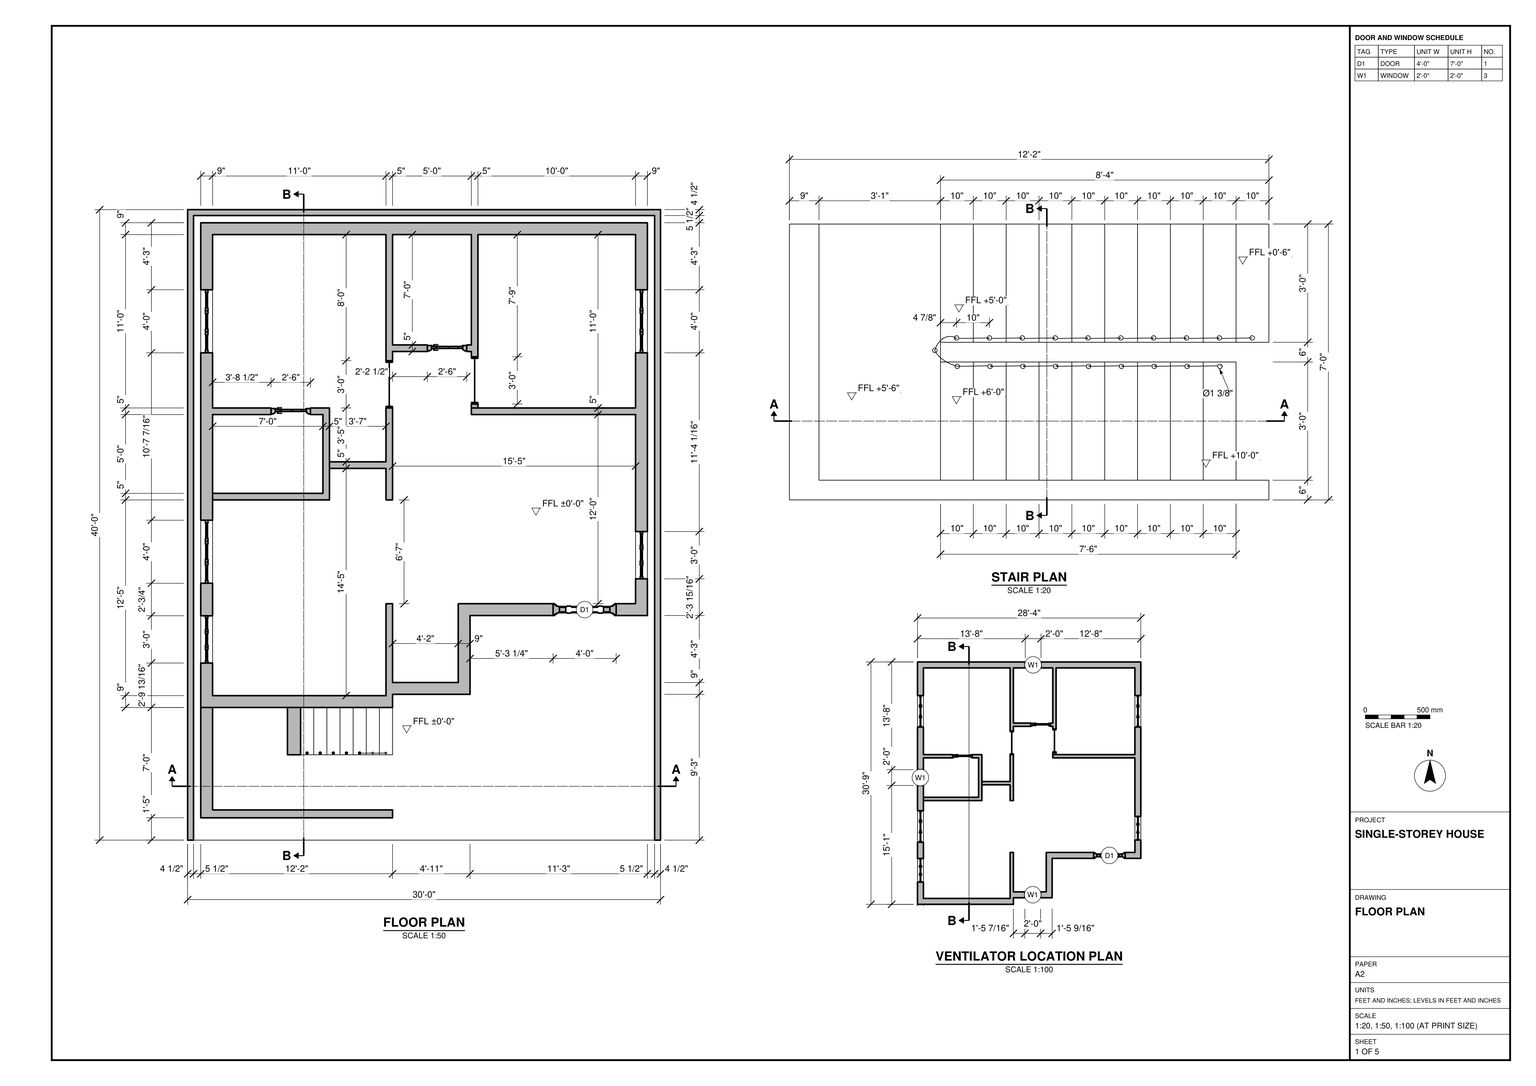
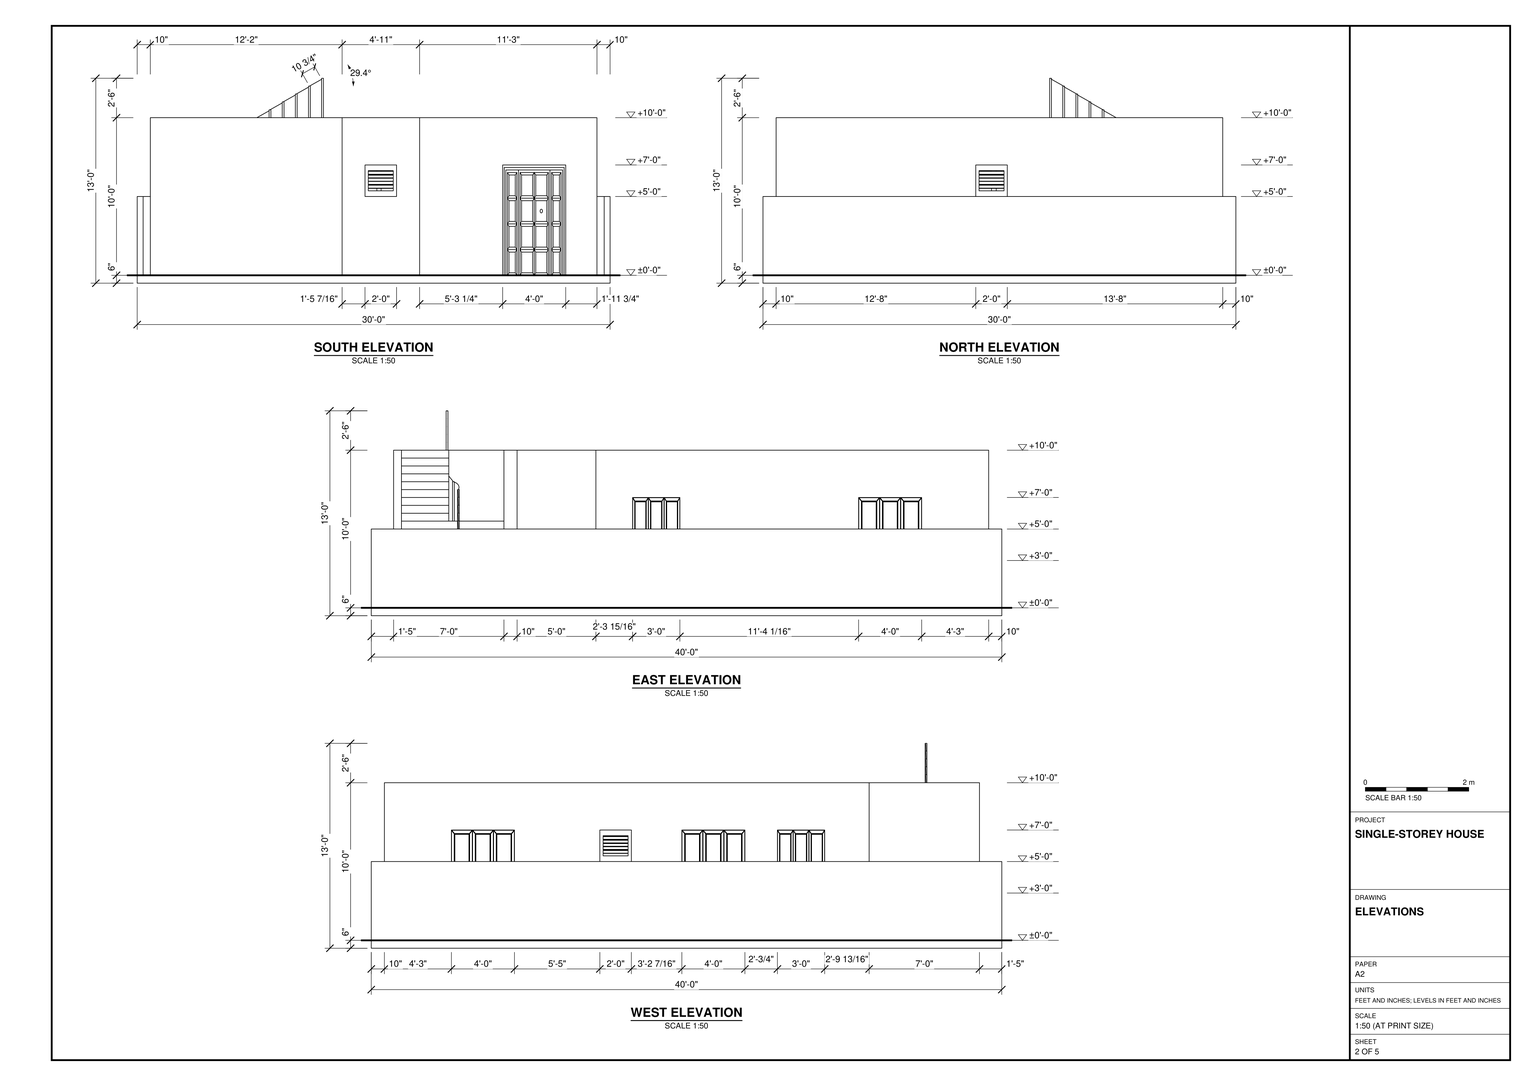
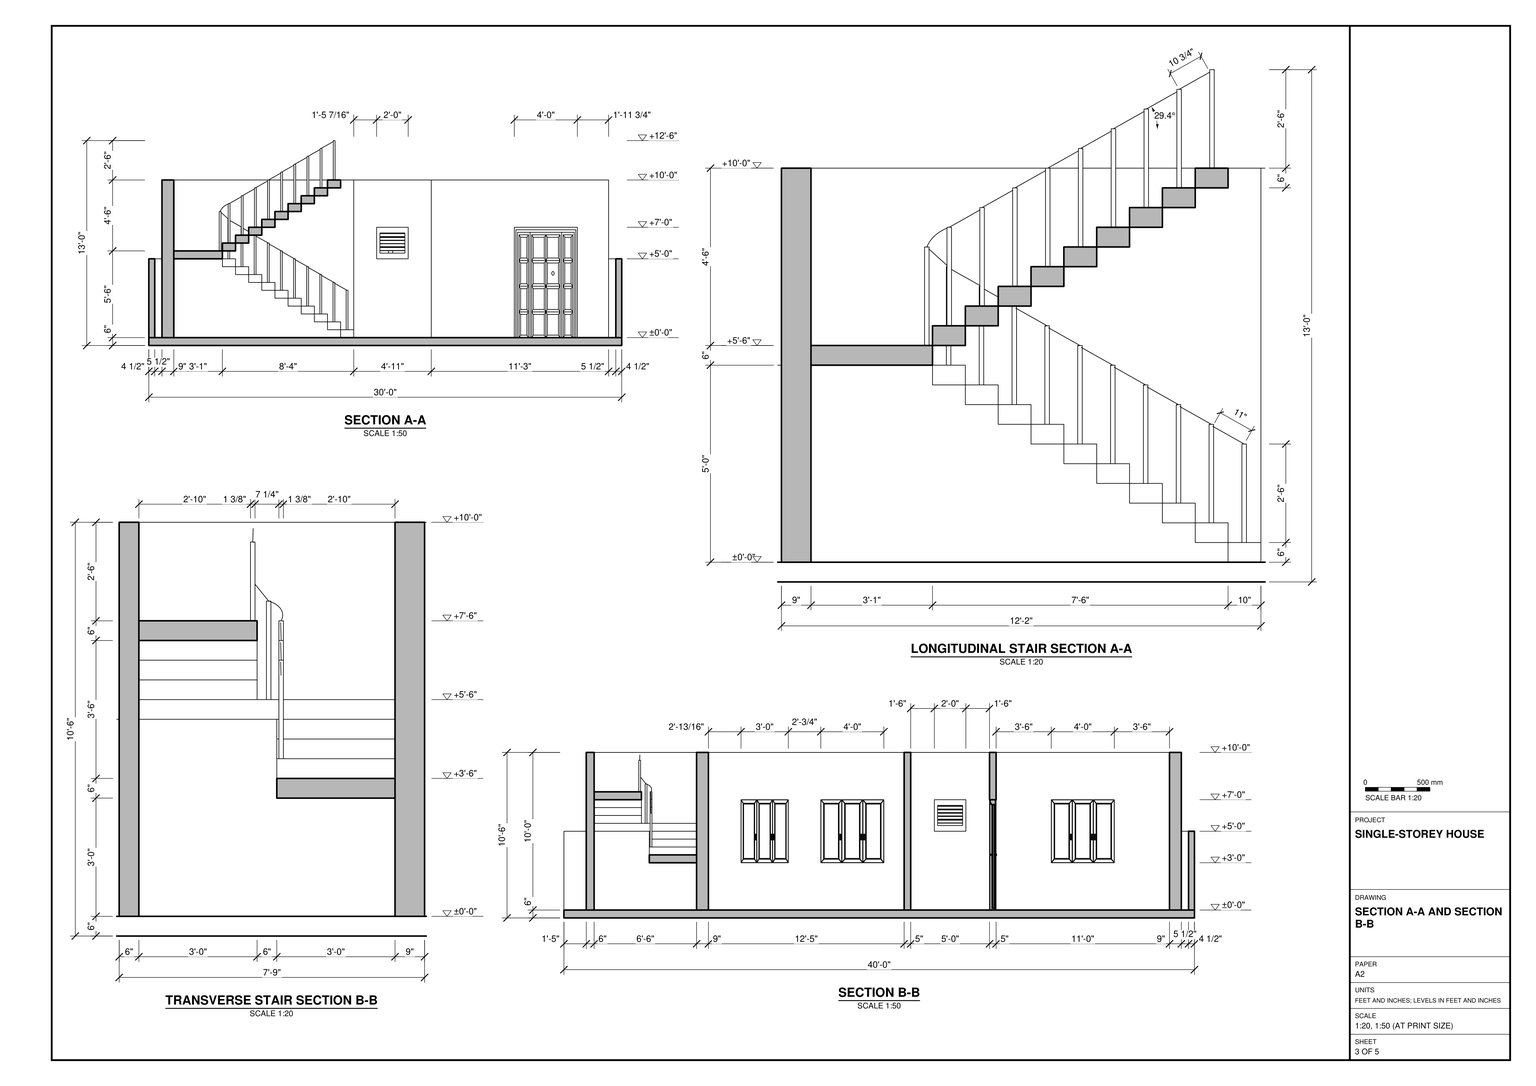
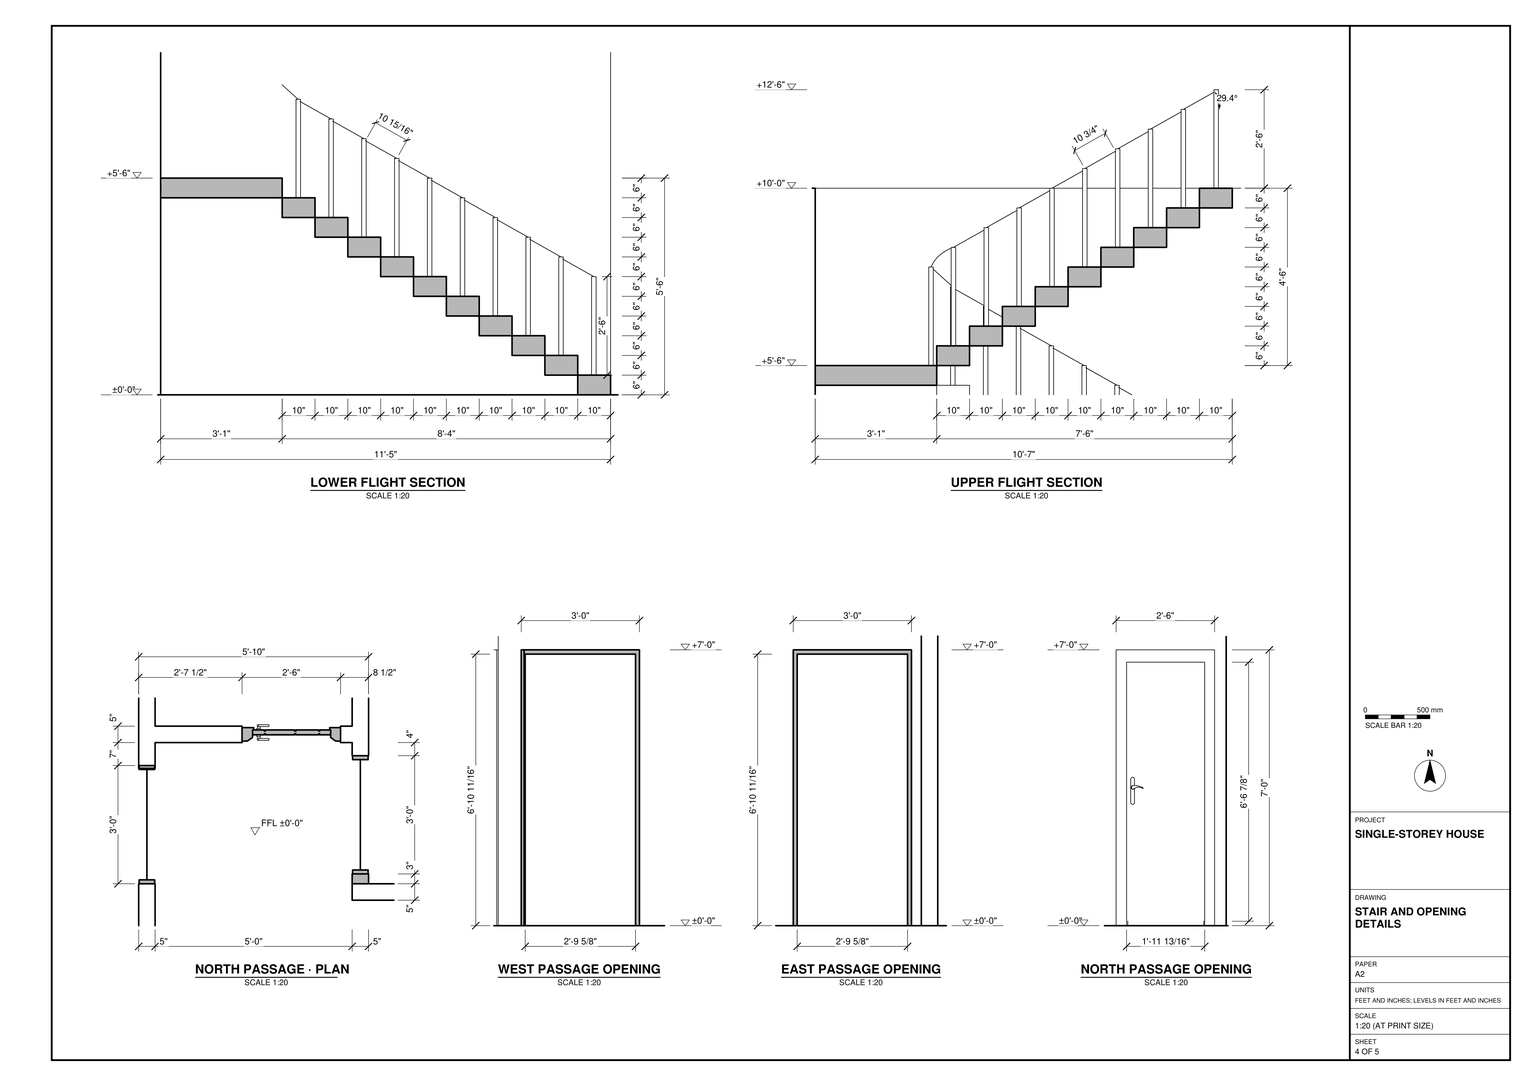
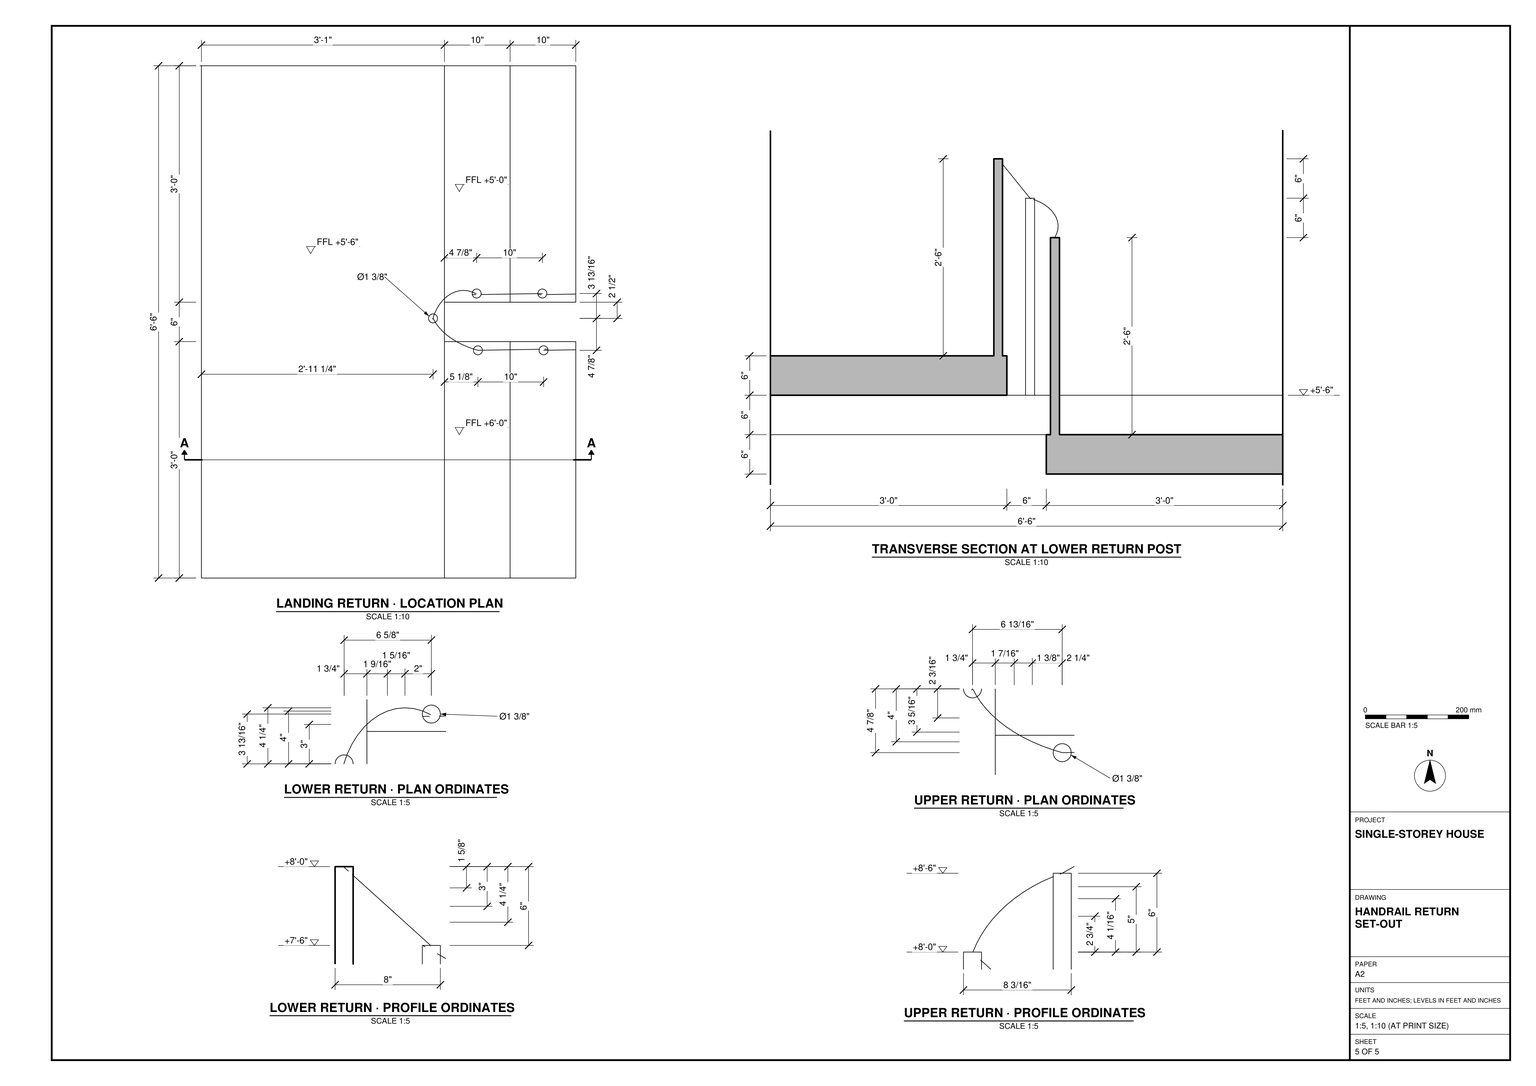
Build the single-storey house in SketchUp from task_files/diagram_01.pdf. Work in feet and inches. Set the ground floor to ±0'-0". The complete model, including the base slab, boundary walls and stair rail, measures 30'-0" along X, 40'-0" along Y and 13'-0" in height.

Use the floor plan to set out the stepped south entrance wall, the rooms and connecting passages, and the open area in front of the house. Follow the drawn wall thicknesses, including the 9" exterior house walls and 5" interior partitions. Extend the base slab beneath the open area and place the lower boundary walls along the sides and rear. Fit the entrance door, framed side windows and high-level louvred windows in their respective openings. Use the ventilator location plan to distinguish the louvred windows from the larger side windows.

Build the external stair to the left of the entrance as viewed from the south. Model both flights, the intermediate landing, individual steps and sloping handrails with upright supports. Keep shell elements and any furniture or joinery pieces in separate groups or components, and use components for repeated parts. Any decor or loose items shown may be suitable library components. Save one SketchUp model as output_files/single_storey_house_with_an_external_return_stair.skp.

# SketchUp Ruby script. Lengths in inches.
U = 1.inch
M = Sketchup.active_model
def pt(a) = Geom::Point3d.new(a.map { |v| v * U })
def face(e, loops, mat)
  f = e.add_face(loops[0].map { |a| pt(a) })
  loops[1..].each { |l| e.add_face(l.map { |a| pt(a) }).erase! }
  f.material = f.back_material = mat if mat
  f
end
# faces: each face lists its corners as indices into pts; further lists are holes
def faces(e, pts, list, mat = nil) = list.each { |f| face(e, (f[0].is_a?(Array) ? f : [f]).map { |l| l.map { |i| pts[i] } }, mat) }
# xy, xz, yz: faces in a plane at the given z, y or x. An outline is a flat list of corners, or four numbers for a rectangle; further outlines are holes
def ring(l) = l.size == 4 ? [[l[0], l[1]], [l[2], l[1]], [l[2], l[3]], [l[0], l[3]]] : l.each_slice(2).to_a
def flat(e, list, mat, &to3) = list.each { |f| face(e, (f[0].is_a?(Array) ? f : [f]).map { |l| ring(l).map { |u, v| to3.(u, v) } }, mat) }
def xy(e, z, list, mat = nil) = flat(e, list, mat) { |x, y| [x, y, z] }
def xz(e, y, list, mat = nil) = flat(e, list, mat) { |x, z| [x, y, z] }
def yz(e, x, list, mat = nil) = flat(e, list, mat) { |y, z| [x, y, z] }
def lines(e, pts, list) = list.each { |a, b| e.add_line(pt(pts[a]), pt(pts[b])) }
# prism: a flat outline (further loops are holes) pulled along v
def prism(e, loops, v, mat = nil)
  f = face(e, loops, mat); d = Geom::Vector3d.new(v.map { |x| x * U })
  f.pushpull(f.normal.samedirection?(d) ? d.length : -d.length)
end
def box(e, o, s, mat = nil) = prism(e, [[o, [o[0] + s[0], o[1], o[2]], [o[0] + s[0], o[1] + s[1], o[2]], [o[0], o[1] + s[1], o[2]]]], [0, 0, s[2]], mat)
def at(x, y, z, deg = 0) = Geom::Transformation.translation(pt([x, y, z])) * Geom::Transformation.rotation(ORIGIN, Z_AXIS, deg.degrees)
def axes(o, x, y, z) = Geom::Transformation.new([*x, 0, *y, 0, *z, 0, *pt(o).to_a, 1])
def part(name) = M.definitions.add(name)
# library, detail: a bought-in or finely detailed component or shape, given as its bounding box
def library(name, o, s) = part(name).tap { |d| box(d.entities, o, s) }
def detail(e, o, s) = box(e.add_group.entities, o, s)
def put(e, d, t, mat = nil) = e.add_instance(d, t).tap { |i| i.material = mat if mat }
def group(e, t, mat = nil) = e.add_group.tap { |g| g.transformation = t; g.material = mat if mat }.entities
root = M.entities
M.materials.add("Polis06_194").color = [79, 50, 36]
M.materials.add("TEAKcrown-cut").color = [186, 122, 55]
M.materials.add("[Translucent_Glass_Gray]3").color = [255, 255, 255]
M.materials["[Translucent_Glass_Gray]3"].alpha = 0.5
c1 = part("Stair landing")
xy(c1.entities,0,[[-27,-42,10,36]])
xy(c1.entities,6,[[-27,-42,10,36]])
xz(c1.entities,-42,[[-27,0,10,6]])
yz(c1.entities,-27,[[-42,0,36,6]])
yz(c1.entities,10,[[-42,0,36,6]])
c2 = part("Tread with baluster")
xy(c2.entities,0,[[0,0,10,36]])
xy(c2.entities,6,[[[0,0,10,36],[4.9,0.64,4.73,0.66,4.5625,0.73,4.42,0.84,4.31,0.98,4.24,1.15,4.22,1.32,4.24,1.5,4.31,1.67,4.42,1.81,4.5625,1.92,4.73,1.99,4.9,2.01,5.08,1.99,5.25,1.92,5.39,1.81,5.5,1.67,5.57,1.5,5.59,1.32,5.57,1.15,5.5,0.98,5.39,0.84,5.25,0.73,5.08,0.66]]])
xy(c2.entities,36,[[4.9,0.64,5.08,0.66,5.25,0.73,5.39,0.84,5.5,0.98,5.57,1.15,5.59,1.32,5.57,1.5,5.5,1.67,5.39,1.81,5.25,1.92,5.08,1.99,4.9,2.01,4.73,1.99,4.5625,1.92,4.42,1.81,4.31,1.67,4.24,1.5,4.22,1.32,4.24,1.15,4.31,0.98,4.42,0.84,4.5625,0.73,4.73,0.66]])
xz(c2.entities,0,[[0,0,10,6]])
xz(c2.entities,36,[[0,0,10,6]])
yz(c2.entities,0,[[0,0,36,6]])
yz(c2.entities,10,[[0,0,36,6]])
p = [[4.73,0.66,6],[4.9,0.64,6],[4.9,0.64,36],[4.73,0.66,36],[5.08,0.66,6],[5.08,0.66,36],
  [4.42,0.84,6],[4.5625,0.73,6],[4.5625,0.73,36],[4.42,0.84,36],[5.25,0.73,6],[5.25,0.73,36],
  [5.39,0.84,6],[5.39,0.84,36],[4.31,0.98,6],[4.31,0.98,36],[5.5,0.98,6],[5.5,0.98,36],
  [4.24,1.15,6],[4.24,1.15,36],[5.57,1.15,6],[5.57,1.15,36],[4.22,1.32,6],[4.22,1.32,36],
  [5.59,1.32,6],[5.59,1.32,36],[4.24,1.5,6],[4.24,1.5,36],[5.57,1.5,6],[5.57,1.5,36],
  [4.31,1.67,6],[4.31,1.67,36],[5.5,1.67,6],[5.5,1.67,36],[4.42,1.81,6],[4.42,1.81,36],
  [5.39,1.81,6],[5.39,1.81,36],[4.5625,1.92,6],[4.5625,1.92,36],[5.25,1.92,6],[5.25,1.92,36],
  [4.73,1.99,6],[4.73,1.99,36],[5.08,1.99,6],[5.08,1.99,36],[4.9,2.01,6],[4.9,2.01,36],
  [4.9,1.32,36],[-5.76,1.15,42]]
faces(c2.entities,p,[[0,1,2,3],[1,4,5,2],[6,7,8,9],[7,0,3,8],[4,10,11,5],[10,12,13,11],[14,6,9,15],[12,16,17,13],
  [18,14,15,19],[16,20,21,17],[22,18,19,23],[20,24,25,21],[26,22,23,27],[24,28,29,25],[30,26,27,31],[28,32,33,29],
  [34,30,31,35],[32,36,37,33],[38,34,35,39],[36,40,41,37],[42,38,39,43],[40,44,45,41],[46,42,43,47],[44,46,47,45]])
lines(c2.entities,p,[[48,49]])
c3 = part("Tread with baluster \#1")
xy(c3.entities,0,[[0,0,10,36]])
xy(c3.entities,6,[[[0,0,10,36],[4.9,0.64,4.73,0.66,4.5625,0.73,4.42,0.84,4.31,0.98,4.24,1.15,4.22,1.32,4.24,1.5,4.31,1.67,4.42,1.81,4.5625,1.92,4.73,1.99,4.9,2.01,5.08,1.99,5.25,1.92,5.39,1.81,5.5,1.67,5.57,1.5,5.59,1.32,5.57,1.15,5.5,0.98,5.39,0.84,5.25,0.73,5.08,0.66]]])
xy(c3.entities,36,[[4.9,0.64,5.08,0.66,5.25,0.73,5.39,0.84,5.5,0.98,5.57,1.15,5.59,1.32,5.57,1.5,5.5,1.67,5.39,1.81,5.25,1.92,5.08,1.99,4.9,2.01,4.73,1.99,4.5625,1.92,4.42,1.81,4.31,1.67,4.24,1.5,4.22,1.32,4.24,1.15,4.31,0.98,4.42,0.84,4.5625,0.73,4.73,0.66]])
xz(c3.entities,0,[[0,0,10,6]])
xz(c3.entities,36,[[0,0,10,6]])
yz(c3.entities,0,[[0,0,36,6]])
yz(c3.entities,10,[[0,0,36,6]])
p = [[4.73,0.66,6],[4.9,0.64,6],[4.9,0.64,36],[4.73,0.66,36],[5.08,0.66,6],[5.08,0.66,36],
  [4.42,0.84,6],[4.5625,0.73,6],[4.5625,0.73,36],[4.42,0.84,36],[5.25,0.73,6],[5.25,0.73,36],
  [5.39,0.84,6],[5.39,0.84,36],[4.31,0.98,6],[4.31,0.98,36],[5.5,0.98,6],[5.5,0.98,36],
  [4.24,1.15,6],[4.24,1.15,36],[5.57,1.15,6],[5.57,1.15,36],[4.22,1.32,6],[4.22,1.32,36],
  [5.59,1.32,6],[5.59,1.32,36],[4.24,1.5,6],[4.24,1.5,36],[5.57,1.5,6],[5.57,1.5,36],
  [4.31,1.67,6],[4.31,1.67,36],[5.5,1.67,6],[5.5,1.67,36],[4.42,1.81,6],[4.42,1.81,36],
  [5.39,1.81,6],[5.39,1.81,36],[4.5625,1.92,6],[4.5625,1.92,36],[5.25,1.92,6],[5.25,1.92,36],
  [4.73,1.99,6],[4.73,1.99,36],[5.08,1.99,6],[5.08,1.99,36],[4.9,2.01,6],[4.9,2.01,36]]
faces(c3.entities,p,[[0,1,2,3],[1,4,5,2],[6,7,8,9],[7,0,3,8],[4,10,11,5],[10,12,13,11],[14,6,9,15],[12,16,17,13],
  [18,14,15,19],[16,20,21,17],[22,18,19,23],[20,24,25,21],[26,22,23,27],[24,28,29,25],[30,26,27,31],[28,32,33,29],
  [34,30,31,35],[32,36,37,33],[38,34,35,39],[36,40,41,37],[42,38,39,43],[40,44,45,41],[46,42,43,47],[44,46,47,45]])
c4 = part("Tread with baluster \#2")
xy(c4.entities,0,[[0,0,10,36]])
xy(c4.entities,6,[[[0,0,10,36],[4.9,0.64,4.73,0.66,4.5625,0.73,4.42,0.84,4.31,0.98,4.24,1.15,4.22,1.32,4.24,1.5,4.31,1.67,4.42,1.81,4.5625,1.92,4.73,1.99,4.9,2.01,5.08,1.99,5.25,1.92,5.39,1.81,5.5,1.67,5.57,1.5,5.59,1.32,5.57,1.15,5.5,0.98,5.39,0.84,5.25,0.73,5.08,0.66]]])
xy(c4.entities,36,[[4.9,0.64,5.08,0.66,5.25,0.73,5.39,0.84,5.5,0.98,5.57,1.15,5.59,1.32,5.57,1.5,5.5,1.67,5.39,1.81,5.25,1.92,5.08,1.99,4.9,2.01,4.73,1.99,4.5625,1.92,4.42,1.81,4.31,1.67,4.24,1.5,4.22,1.32,4.24,1.15,4.31,0.98,4.42,0.84,4.5625,0.73,4.73,0.66]])
xz(c4.entities,0,[[0,0,10,6]])
xz(c4.entities,36,[[0,0,10,6]])
yz(c4.entities,0,[[0,0,36,6]])
yz(c4.entities,10,[[0,0,36,6]])
p = [[4.73,0.66,6],[4.9,0.64,6],[4.9,0.64,36],[4.73,0.66,36],[5.08,0.66,6],[5.08,0.66,36],
  [4.42,0.84,6],[4.5625,0.73,6],[4.5625,0.73,36],[4.42,0.84,36],[5.25,0.73,6],[5.25,0.73,36],
  [5.39,0.84,6],[5.39,0.84,36],[4.31,0.98,6],[4.31,0.98,36],[5.5,0.98,6],[5.5,0.98,36],
  [4.24,1.15,6],[4.24,1.15,36],[5.57,1.15,6],[5.57,1.15,36],[4.22,1.32,6],[4.22,1.32,36],
  [5.59,1.32,6],[5.59,1.32,36],[4.24,1.5,6],[4.24,1.5,36],[5.57,1.5,6],[5.57,1.5,36],
  [4.31,1.67,6],[4.31,1.67,36],[5.5,1.67,6],[5.5,1.67,36],[4.42,1.81,6],[4.42,1.81,36],
  [5.39,1.81,6],[5.39,1.81,36],[4.5625,1.92,6],[4.5625,1.92,36],[5.25,1.92,6],[5.25,1.92,36],
  [4.73,1.99,6],[4.73,1.99,36],[5.08,1.99,6],[5.08,1.99,36],[4.9,2.01,6],[4.9,2.01,36]]
faces(c4.entities,p,[[0,1,2,3],[1,4,5,2],[6,7,8,9],[7,0,3,8],[4,10,11,5],[10,12,13,11],[14,6,9,15],[12,16,17,13],
  [18,14,15,19],[16,20,21,17],[22,18,19,23],[20,24,25,21],[26,22,23,27],[24,28,29,25],[30,26,27,31],[28,32,33,29],
  [34,30,31,35],[32,36,37,33],[38,34,35,39],[36,40,41,37],[42,38,39,43],[40,44,45,41],[46,42,43,47],[44,46,47,45]])
c5 = library("Door",[0,0,0],[79.98,10,87.99])
c6 = part("Flush door")
xy(c6.entities,0,[[0,0,4.72,1.18],[0,34.25,4.72,35.43]],"Polis06_194")
xy(c6.entities,85.26,[[0,1.18,4.72,34.25]],"Polis06_194")
xy(c6.entities,86.61,[[0,0,4.72,35.43]],"Polis06_194")
xz(c6.entities,0,[[0,0,4.72,86.61]],"Polis06_194")
xz(c6.entities,1.18,[[0,0,2.36,85.26],[2.36,0,4.72,85.26]],"Polis06_194")
xz(c6.entities,34.25,[[0,0,4.72,85.26]],"Polis06_194")
xz(c6.entities,35.43,[[0,0,4.72,86.61]],"Polis06_194")
yz(c6.entities,0,[[0,0,1.18,86.61],[34.25,0,35.43,86.61],[1.18,85.26,34.25,86.61]],"Polis06_194")
yz(c6.entities,2.36,[[1.18,0,34.25,0,34.25,85.21,1.18,85.26]],"Polis06_194")
yz(c6.entities,4.72,[[0,0,1.18,86.61],[34.25,0,35.43,86.61],[1.18,85.26,34.25,86.61]],"Polis06_194")
c7 = library("Untitled",[0,0,-0.0625],[52.25,7.08,114.54])
c8 = library("Three-panel window",[0,0,0],[5.02,84.63,60])
c9 = library("Three-panel window \#1",[0,0,0],[5.02,84.63,60])
c10 = part("Component\#16")
box(c10.entities,[0,0,0],[19,0.25,3.7],"[Translucent_Glass_Gray]3")
c11 = part("Ventilation_window")
g1 = group(c11.entities,at(-76.91,6.38,0),"TEAKcrown-cut")
xy(g1,-1.7,[[0,0,24,3]])
xy(g1,2.5,[[2.5,0,21.5,3]])
xy(g1,17.5,[[2.5,0,21.5,3]])
xy(g1,21.7,[[0,0,24,3]])
xz(g1,0,[[[0,-1.7,24,21.7],[2.5,2.5,21.5,17.5]]],"TEAKcrown-cut")
xz(g1,3,[[[0,-1.7,24,21.7],[2.5,2.5,21.5,17.5]]])
yz(g1,0,[[0,-1.7,3,21.7]])
yz(g1,2.5,[[0,2.5,3,2.5,3,4.31,0,6.48],[3,4.31,3,17.5,0,17.5,0,6.48]])
yz(g1,21.5,[[0,2.5,3,17.5]])
yz(g1,24,[[0,-1.7,3,21.7]])
put(g1,c10,axes([2.5,3.14,11.94],[1,0,0],[0,0.58779,0.80902],[0,-0.80902,0.58779]))
put(g1,c10,axes([2.5,3.16,14.6],[1,0,0],[0,0.58779,0.80902],[0,-0.80902,0.58779]))
put(g1,c10,axes([2.5,3,4.31],[1,0,0],[0,0.58779,0.80902],[0,-0.80902,0.58779]))
put(g1,c10,axes([2.5,3.14,9.46],[1,0,0],[0,0.58779,0.80902],[0,-0.80902,0.58779]))
put(g1,c10,axes([2.5,2.99,7.08],[1,0,0],[0,0.58779,0.80902],[0,-0.80902,0.58779]))
c12 = part("ventilator")
put(c12.entities,c11,axes([8.375,-1.09,0.54],[0.09843,0,0],[0,0.09,0],[0,0,0.08412]))
c13 = part("Group2\#1")
xy(c13.entities,0,[[149.12,170.58,149.12,179.58,281.12,179.58,281.12,249.58,286.12,249.58,286.12,189.58,336.12,189.58,336.12,249.58,408.34,249.58,408.34,240.58,345.12,240.58,345.12,180.58,286.12,180.58,286.12,170.58],[140.12,179.58,140.12,539.58,480.12,539.58,480.12,240.58,456.34,240.58,456.34,249.58,471.12,249.58,471.12,393.58,346.12,393.58,346.12,398.58,471.12,398.58,471.12,530.58,351.12,530.58,351.12,437.58,346.12,437.58,346.12,441.58,342.59,441.58,342.59,446.58,346.12,446.58,346.12,530.58,286.12,530.58,286.12,446.58,312.59,446.58,312.59,441.58,286.12,441.58,286.12,433.71,281.12,433.71,281.12,530.58,149.12,530.58,149.12,398.58,193.62,398.58,193.62,393.58,149.12,393.58,149.12,179.58],[149.12,328.58,149.12,333.58,233.12,333.58,233.12,393.58,223.62,393.58,223.62,398.58,238.12,398.58,238.12,328.58],[281.12,328.58,281.12,352.58,238.12,352.58,238.12,357.58,281.12,357.58,281.12,398.58,286.12,398.58,286.12,328.58],[346.12,398.58,351.12,401.58]])
xy(c13.entities,36,[[140.12,204.4,149.12,240.4],[140.12,265.15,149.12,313.15],[471.12,268.52,480.12,304.52],[140.12,440.58,149.12,488.58],[471.12,440.58,480.12,488.58]])
xy(c13.entities,60,[[303.55,180.58,327.55,189.58],[140.12,351.58,149.12,375.58],[304.13,530.58,328.13,539.58]])
xy(c13.entities,84,[[303.55,180.58,327.55,189.58],[140.12,204.4,149.12,240.4],[408.34,240.58,456.34,249.58],[140.12,265.15,149.12,313.15],[471.12,268.52,480.12,304.52],
  [140.12,351.58,149.12,375.58],[193.62,393.58,223.62,398.58],[281.12,398.58,286.12,433.71],[346.12,401.58,351.12,437.58],[140.12,440.58,149.12,488.58],
  [471.12,440.58,480.12,488.58],[312.59,441.58,342.59,446.58],[304.13,530.58,328.13,539.58]])
xy(c13.entities,120,[[[140.12,170.58,286.12,170.58,286.12,180.58,345.12,180.58,345.12,240.58,480.12,240.58,480.12,539.58,140.12,539.58],[149.12,179.58,149.12,393.58,233.12,393.58,233.12,333.58,149.12,333.58,149.12,328.58,238.12,328.58,238.12,398.58,149.12,398.58,149.12,530.58,281.12,530.58,281.12,357.58,238.12,357.58,238.12,352.58,281.12,352.58,281.12,328.58,286.12,328.58,286.12,441.58,346.12,441.58,346.12,398.58,351.12,398.58,351.12,530.58,471.12,530.58,471.12,398.58,346.12,398.58,346.12,393.58,471.12,393.58,471.12,249.58,336.12,249.58,336.12,189.58,286.12,189.58,286.12,249.58,281.12,249.58,281.12,179.58],[286.12,446.58,346.12,530.58]]])
xz(c13.entities,170.58,[[140.12,0,286.12,120]])
xz(c13.entities,179.58,[[149.12,0,281.12,120]])
xz(c13.entities,180.58,[[[286.12,0,345.12,120],[303.55,60,327.55,84]]])
xz(c13.entities,189.58,[[[286.12,0,336.12,120],[303.55,60,327.55,84]]])
xz(c13.entities,204.4,[[140.12,36,149.12,84]])
xz(c13.entities,240.4,[[140.12,36,149.12,84]])
xz(c13.entities,240.58,[[345.12,0,408.34,0,408.34,84,456.34,84,456.34,0,480.12,0,480.12,120,345.12,120]])
xz(c13.entities,249.58,[[281.12,0,286.12,120],[336.12,0,336.12,120,471.12,120,471.12,0,456.34,0,456.34,84,408.34,84,408.34,0]])
xz(c13.entities,265.15,[[140.12,36,149.12,84]])
xz(c13.entities,268.52,[[471.12,36,480.12,84]])
xz(c13.entities,304.52,[[471.12,36,480.12,84]])
xz(c13.entities,313.15,[[140.12,36,149.12,84]])
xz(c13.entities,328.58,[[149.12,0,238.12,120],[281.12,0,286.12,120]])
xz(c13.entities,333.58,[[149.12,0,233.12,120]])
xz(c13.entities,351.58,[[140.12,60,149.12,84]])
xz(c13.entities,352.58,[[238.12,0,281.12,120]])
xz(c13.entities,357.58,[[238.12,0,281.12,120]])
xz(c13.entities,375.58,[[140.12,60,149.12,84]])
xz(c13.entities,393.58,[[149.12,0,193.62,0,193.62,84,223.62,84,223.62,0,233.12,0,233.12,120,149.12,120],[346.12,0,471.12,120]])
xz(c13.entities,398.58,[[149.12,0,149.12,120,238.12,120,238.12,0,223.62,0,223.62,84,193.62,84,193.62,0],[281.12,0,286.12,84],[346.12,0,351.12,120],[351.12,0,471.12,120]])
xz(c13.entities,401.58,[[346.12,0,351.12,84]])
xz(c13.entities,433.71,[[281.12,0,286.12,84]])
xz(c13.entities,437.58,[[346.12,0,351.12,84]])
xz(c13.entities,440.58,[[140.12,36,149.12,84],[471.12,36,480.12,84]])
xz(c13.entities,441.58,[[286.12,0,312.59,0,312.59,84,342.59,84,342.59,0,346.12,0,346.12,120,286.12,120]])
xz(c13.entities,446.58,[[286.12,0,286.12,120,346.12,120,346.12,0,342.59,0,342.59,84,312.59,84,312.59,0]])
xz(c13.entities,488.58,[[140.12,36,149.12,84],[471.12,36,480.12,84]])
xz(c13.entities,530.58,[[149.12,0,281.12,120],[[286.12,0,346.12,120],[304.13,60,328.13,84]],[351.12,0,471.12,120]])
xz(c13.entities,539.58,[[[140.12,0,480.12,120],[304.13,60,328.13,84]]])
yz(c13.entities,140.12,[[[170.58,0,539.58,120],[440.58,36,488.58,84],[265.15,36,313.15,84],[204.4,36,240.4,84],[351.58,60,375.58,84]]])
yz(c13.entities,149.12,[[[179.58,0,328.58,120],[265.15,36,313.15,84],[204.4,36,240.4,84]],[328.58,0,333.58,120],[[333.58,0,393.58,120],[351.58,60,375.58,84]],[[398.58,0,530.58,120],[440.58,36,488.58,84]]])
yz(c13.entities,193.62,[[393.58,0,398.58,84]])
yz(c13.entities,223.62,[[393.58,0,398.58,84]])
yz(c13.entities,233.12,[[333.58,0,393.58,120]])
yz(c13.entities,238.12,[[328.58,0,352.58,120],[352.58,0,357.58,120],[357.58,0,398.58,120]])
yz(c13.entities,281.12,[[179.58,0,249.58,120],[328.58,0,352.58,120],[357.58,0,357.58,120,530.58,120,530.58,0,433.71,0,433.71,84,398.58,84,398.58,0]])
yz(c13.entities,286.12,[[170.58,0,180.58,120],[189.58,0,249.58,120],[328.58,0,398.58,0,398.58,84,433.71,84,433.71,0,441.58,0,441.58,120,328.58,120],[446.58,0,530.58,120]])
yz(c13.entities,303.55,[[180.58,60,189.58,84]])
yz(c13.entities,304.13,[[530.58,60,539.58,84]])
yz(c13.entities,312.59,[[441.58,0,446.58,84]])
yz(c13.entities,327.55,[[180.58,60,189.58,84]])
yz(c13.entities,328.13,[[530.58,60,539.58,84]])
yz(c13.entities,336.12,[[189.58,0,249.58,120]])
yz(c13.entities,342.59,[[441.58,0,446.58,84]])
yz(c13.entities,345.12,[[180.58,0,240.58,120]])
yz(c13.entities,346.12,[[393.58,0,398.58,120],[398.58,0,398.58,120,441.58,120,441.58,0,437.58,0,437.58,84,401.58,84,401.58,0],[446.58,0,530.58,120]])
yz(c13.entities,351.12,[[398.58,0,401.58,0,401.58,84,437.58,84,437.58,0,530.58,0,530.58,120,398.58,120]])
yz(c13.entities,408.34,[[240.58,0,249.58,84]])
yz(c13.entities,456.34,[[240.58,0,249.58,84]])
yz(c13.entities,471.12,[[[249.58,0,393.58,120],[268.52,36,304.52,84]],[[398.58,0,530.58,120],[440.58,36,488.58,84]]])
yz(c13.entities,480.12,[[[240.58,0,539.58,120],[440.58,36,488.58,84],[268.52,36,304.52,84]]])
prism(root,[[[53.78,63.02,66],[53.92,63.125,66],[54.09,63.19,66],[54.27,63.22,66],[54.44,63.19,66],[54.61,63.125,66],[54.75,63.02,66],[54.86,62.875,66],[54.93,62.71,66],[54.95,62.53,66],[54.93,62.35,66],[54.86,62.1875,66],[54.75,62.04,66],[54.61,61.94,66],[54.44,61.87,66],[54.27,61.84,66],[54.09,61.87,66],[53.92,61.94,66],[53.78,62.04,66],[53.67,62.1875,66],[53.6,62.35,66],[53.58,62.53,66],[53.6,62.71,66],[53.67,62.875,66]]],[0,0,30])
xy(root,0,[[0,0,0,480,360,480,360,0,355.5,0,355.5,475.5,4.5,475.5,4.5,0],[[4.5,0,355.5,475.5],[151,364.125,151,461,19,461,19,419,10,419,10,470,174.01,470,174.01,461,156,461,156,377,182.47,377,182.47,372,156,372,156,364.125],[216,368,216,372,212.47,372,212.47,377,216,377,216,461,198.01,461,198.01,470,350,470,350,419,341,419,341,461,221,461,221,368],[341,234.9375,341,324,216,324,216,329,341,329,341,371,350,371,350,234.9375],[10,17,10,101,19,101,19,23,156,23,156,17],[151,259,151,283,108,283,108,288,151,288,151,329,156,329,156,259],[326.22,171,326.22,180,341,180,341,198.9375,350,198.9375,350,171],[10,243.5625,19,282],[10,110,19,134.82],[10,170.82,19,195.5625]],[10,17,156,17,156,23,19,23,19,101,10,101],[10,101,19,110],[10,110,19,134.82],
  [10,170.82,19,195.5625],[326.22,171,350,171,350,198.9375,341,198.9375,341,180,326.22,180],[341,234.9375,350,234.9375,350,371,341,371,341,329,216,329,216,324,341,324],[10,243.5625,19,282],[151,259,156,259,156,329,151,329,151,288,108,288,108,283,151,283],
  [216,329,221,332],[151,364.125,156,364.125,156,372,182.47,372,182.47,377,156,377,156,461,174.01,461,174.01,470,10,470,10,419,19,419,19,461,151,461],[216,368,221,368,221,461,341,461,341,419,350,419,350,470,198.01,470,198.01,461,216,461,216,377,212.47,377,212.47,372,216,372]])
xy(root,60,[[0,0,4.5,0,4.5,475.5,355.5,475.5,355.5,0,360,0,360,480,0,480]])
xy(root,120,[[10,17,156,17,156,23,19,23,19,101,10,101]])
xz(root,0,[[0,0,4.5,60],[355.5,0,360,60]])
xz(root,17,[[10,0,156,120]])
xz(root,23,[[19,0,156,120]])
xz(root,101,[[10,0,19,120],[146,0,156,6]])
xz(root,475.5,[[4.5,0,355.5,60]])
xz(root,480,[[0,0,360,60]])
yz(root,0,[[0,0,480,60]])
yz(root,4.5,[[0,0,475.5,60]])
yz(root,10,[[17,0,101,120]])
yz(root,19,[[23,0,101,120]])
yz(root,156,[[17,0,23,120]])
yz(root,355.5,[[0,0,475.5,60]])
yz(root,360,[[0,0,480,60]])
p = [[108,259,0],[108,283,0],[10,306,0],[10,371,0],[19,259,0],[19,264,0],
  [103,264,0],[103,324,0],[19,324,0],[19,306,0],[206,180,0],[206,120,0],
  [19,101,0],[146,101,0],[215,171,0],[215,111,0],[278.22,171,0],[151,180,0],
  [156,180,0],[156,120,0],[151,110,0],[19,110,0],[156,111,0],[156,101,0],
  [108,288,0],[108,329,0],[19,371,0],[19,329,0],[278.22,180,0],[60.85,66.28,90],
  [60.21,66.57,90.57],[59.56,66.75,91.17],[58.89,66.8,91.78],[58.22,66.74,92.38],[57.56,66.55,92.97],[56.93,66.25,93.55],
  [56.33,65.84,94.09],[55.78,65.32,94.58],[55.28,64.71,95.03],[54.85,64.02,95.42],[54.49,63.25,95.75],[54.21,62.43,96],
  [54.29,62.52,96],[54.58,61.99,96.65],[54.92,61.48,97.28],[55.32,60.99,97.9],[55.78,60.51,98.49],[56.29,60.06,99.05],
  [56.85,59.63,99.58],[57.46,59.23,100.08],[58.11,58.85,100.54],[58.8,58.51,100.97],[59.54,58.2,101.35],[60.3,57.92,101.7],
  [61.1,57.68,102]]
lines(root,p,[[0,1],[2,3],[4,0],[5,6],[6,7],[8,9],[10,11],[12,13],[14,15],[14,16],[17,18],[18,19],
  [20,21],[20,17],[22,23],[24,25],[3,26],[26,27],[9,2],[16,28],[28,10],[29,30],[30,31],[31,32],
  [32,33],[33,34],[34,35],[35,36],[36,37],[37,38],[38,39],[39,40],[40,41],[42,43],[43,44],[44,45],
  [45,46],[46,47],[47,48],[48,49],[49,50],[50,51],[51,52],[52,53],[53,54]])
put(root,c1,at(46,65,60))
put(root,c2,at(116,65,18))
put(root,c2,at(136,65,6))
put(root,c2,at(146,65,0))
put(root,c2,at(126,65,12))
put(root,c2,at(76,65,42))
put(root,c3,at(56,65,54))
put(root,c2,at(106,65,24))
put(root,c2,at(66,65,48))
put(root,c2,at(96,65,30))
put(root,c2,at(86,65,36))
put(root,c2,at(106,59,90,180))
put(root,c2,at(76,59,72,180))
put(root,c4,at(146,59,114,180))
put(root,c2,at(136,59,108,180))
put(root,c2,at(116,59,96,180))
put(root,c2,at(96,59,84,180))
put(root,c2,at(126,59,102,180))
put(root,c2,at(66,59,66,180))
put(root,c2,at(86,59,78,180))
put(root,c5,axes([278.22,171,0],[0.60018,0,0],[0,0.9,0],[0,0,0.95467]))
put(root,c6,axes([151.14,365,0],[1,0,0],[0,-1.016,0],[0,0,0.96982]))
put(root,c6,axes([216.14,368,0],[1,0,0],[0,-1.016,0],[0,0,0.96982]))
put(root,c7,axes([182.47,372.45,0.05],[0.57416,0,0],[0,0.706,0],[0,0,0.73337]))
put(root,c7,axes([63.5,324.45,0.05],[0.57416,0,0],[0,0.706,0],[0,0,0.73337]))
put(root,c8,axes([342.99,371,36],[1,0,0],[0,0.56717,0],[0,0,0.8]))
put(root,c8,axes([11.99,195.5625,36],[1,0,0],[0,0.56717,0],[0,0,0.8]))
put(root,c8,axes([11.99,371,36],[1,0,0],[0,0.56717,0],[0,0,0.8]))
put(root,c9,axes([342.99,198.9375,36],[1,0,0],[0,0.42538,0],[0,0,0.8]))
put(root,c9,axes([11.99,134.82,36],[1,0,0],[0,0.42538,0],[0,0,0.8]))
put(root,c12,axes([165.84,469.38,55.2],[10.16,0,0],[0,10.07748,0],[0,0,12.192]))
put(root,c12,axes([10.62,273.83,55.2],[0,10.16,0],[-10.07748,0,0],[0,0,12.192]))
put(root,c12,axes([165.26,111.9,55.2],[10.16,0,0],[0,-10.07748,0],[0,0,12.192]))
g2 = group(root,at(0,0,-6))
box(g2,[0,0,0],[360,480,6])
put(root,c13,at(-130.12,-69.58,0))
